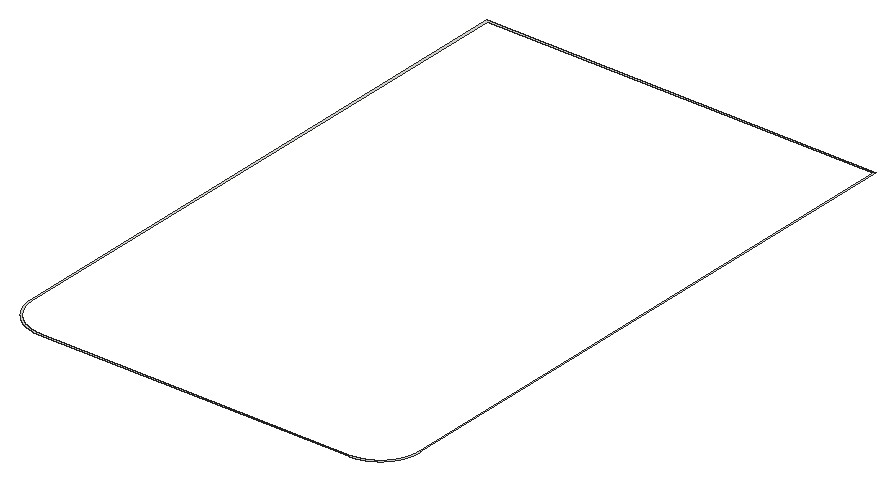
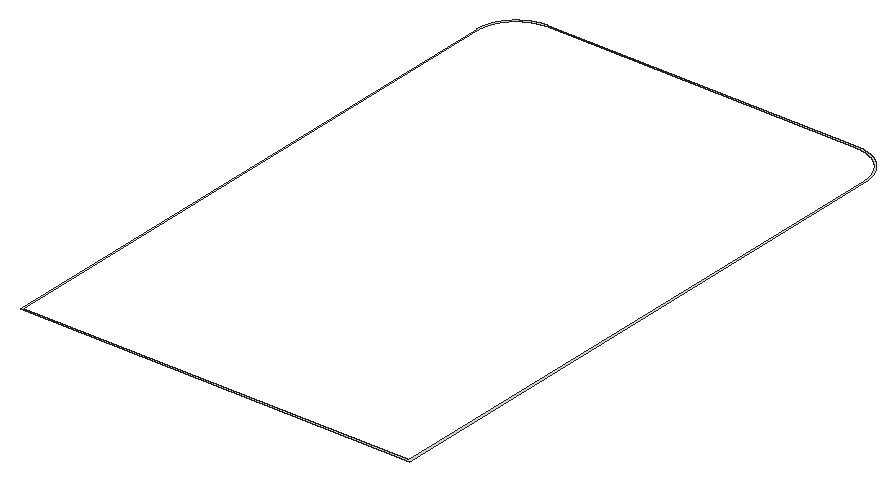
# SketchUp Ruby script. Lengths in inches.
U = 1.inch
M = Sketchup.active_model
def pt(a) = Geom::Point3d.new(a.map { |v| v * U })
def face(e, loops, mat)
  f = e.add_face(loops[0].map { |a| pt(a) })
  loops[1..].each { |l| e.add_face(l.map { |a| pt(a) }).erase! }
  f.material = f.back_material = mat if mat
  f
end
# faces: each face lists its corners as indices into pts; further lists are holes
def faces(e, pts, list, mat = nil) = list.each { |f| face(e, (f[0].is_a?(Array) ? f : [f]).map { |l| l.map { |i| pts[i] } }, mat) }
# xy, xz, yz: faces in a plane at the given z, y or x. An outline is a flat list of corners, or four numbers for a rectangle; further outlines are holes
def ring(l) = l.size == 4 ? [[l[0], l[1]], [l[2], l[1]], [l[2], l[3]], [l[0], l[3]]] : l.each_slice(2).to_a
def flat(e, list, mat, &to3) = list.each { |f| face(e, (f[0].is_a?(Array) ? f : [f]).map { |l| ring(l).map { |u, v| to3.(u, v) } }, mat) }
def xy(e, z, list, mat = nil) = flat(e, list, mat) { |x, y| [x, y, z] }
def xz(e, y, list, mat = nil) = flat(e, list, mat) { |x, z| [x, y, z] }
def yz(e, x, list, mat = nil) = flat(e, list, mat) { |y, z| [x, y, z] }
def lines(e, pts, list) = list.each { |a, b| e.add_line(pt(pts[a]), pt(pts[b])) }
# prism: a flat outline (further loops are holes) pulled along v
def prism(e, loops, v, mat = nil)
  f = face(e, loops, mat); d = Geom::Vector3d.new(v.map { |x| x * U })
  f.pushpull(f.normal.samedirection?(d) ? d.length : -d.length)
end
def box(e, o, s, mat = nil) = prism(e, [[o, [o[0] + s[0], o[1], o[2]], [o[0] + s[0], o[1] + s[1], o[2]], [o[0], o[1] + s[1], o[2]]]], [0, 0, s[2]], mat)
def at(x, y, z, deg = 0) = Geom::Transformation.translation(pt([x, y, z])) * Geom::Transformation.rotation(ORIGIN, Z_AXIS, deg.degrees)
def axes(o, x, y, z) = Geom::Transformation.new([*x, 0, *y, 0, *z, 0, *pt(o).to_a, 1])
def part(name) = M.definitions.add(name)
# library, detail: a bought-in or finely detailed component or shape, given as its bounding box
def library(name, o, s) = part(name).tap { |d| box(d.entities, o, s) }
def detail(e, o, s) = box(e.add_group.entities, o, s)
def put(e, d, t, mat = nil) = e.add_instance(d, t).tap { |i| i.material = mat if mat }
def group(e, t, mat = nil) = e.add_group.tap { |g| g.transformation = t; g.material = mat if mat }.entities
root = M.entities
xy(root,349.5,[[[38.61,204,270.39,204,270.79,204.01,271.18,204.02,271.57,204.04,271.96,204.0625,272.35,204.09,272.75,204.125,273.14,204.16,273.92,204.26,274.3,204.31,275.08,204.43,275.47,204.5,275.85,204.58,276.24,204.66,276.62,204.74,277.38,204.92,277.76,205.02,278.14,205.125,278.52,205.24,278.9,205.35,279.64,205.59,280.38,205.85,280.75,205.99,281.12,206.14,281.48,206.28,281.84,206.4375,282.2,206.59,282.56,206.76,282.92,206.92,283.27,207.09,283.97,207.45,284.31,207.64,284.66,207.83,285,208.02,285.34,208.22,285.67,208.42,286.01,208.63,286.34,208.84,286.67,209.06,286.99,209.28,287.3125,209.5,287.63,209.73,287.95,209.96,288.57,210.44,288.88,210.6875,289.18,210.93,289.48,211.1875,289.78,211.44,290.07,211.71,290.36,211.97,290.65,212.24,290.93,212.51,291.49,213.07,291.76,213.35,292.03,213.64,292.29,213.93,292.56,214.22,292.8125,214.52,293.07,214.82,293.3125,215.12,293.56,215.43,294.04,216.05,294.27,216.37,294.5,216.6875,294.72,217.01,294.94,217.33,295.16,217.66,295.37,217.99,295.58,218.33,295.78,218.66,295.98,219,296.17,219.34,296.36,219.69,296.55,220.03,296.91,220.73,297.08,221.08,297.24,221.44,297.41,221.8,297.5625,222.16,297.72,222.52,297.86,222.88,298.01,223.25,298.15,223.62,298.41,224.36,298.65,225.1,298.76,225.48,298.875,225.86,298.98,226.24,299.08,226.62,299.26,227.38,299.34,227.76,299.42,228.15,299.5,228.53,299.57,228.92,299.69,229.7,299.74,230.08,299.84,230.86,299.875,231.25,299.91,231.65,299.9375,232.04,299.96,232.43,299.98,232.82,299.99,233.21,300,233.61,300,660,9,660,9,233.61,9.01,233.21,9.02,232.82,9.04,232.43,9.0625,232.04,9.09,231.65,9.125,231.25,9.16,230.86,9.26,230.08,9.31,229.7,9.43,228.92,9.5,228.53,9.58,228.15,9.66,227.76,9.74,227.38,9.92,226.62,10.02,226.24,10.125,225.86,10.24,225.48,10.35,225.1,10.59,224.36,10.85,223.62,10.99,223.25,11.14,222.88,11.28,222.52,11.4375,222.16,11.59,221.8,11.76,221.44,11.92,221.08,12.09,220.73,12.45,220.03,12.64,219.69,12.83,219.34,13.02,219,13.22,218.66,13.42,218.33,13.63,217.99,13.84,217.66,14.06,217.33,14.28,217.01,14.5,216.6875,14.73,216.37,14.96,216.05,15.44,215.43,15.6875,215.12,15.93,214.82,16.1875,214.52,16.44,214.22,16.71,213.93,16.97,213.64,17.24,213.35,17.51,213.07,18.07,212.51,18.35,212.24,18.64,211.97,18.93,211.71,19.22,211.44,19.52,211.1875,19.82,210.93,20.12,210.6875,20.43,210.44,21.05,209.96,21.37,209.73,21.6875,209.5,22.01,209.28,22.33,209.06,22.66,208.84,22.99,208.63,23.33,208.42,23.66,208.22,24,208.02,24.34,207.83,24.69,207.64,25.03,207.45,25.73,207.09,26.08,206.92,26.44,206.76,26.8,206.59,27.16,206.4375,27.52,206.28,27.88,206.14,28.25,205.99,28.62,205.85,29.36,205.59,30.1,205.35,30.48,205.24,30.86,205.125,31.24,205.02,31.62,204.92,32.38,204.74,32.76,204.66,33.15,204.58,33.53,204.5,33.92,204.43,34.7,204.31,35.08,204.26,35.86,204.16,36.25,204.125,36.65,204.09,37.04,204.0625,37.43,204.04,37.82,204.02,38.21,204.01],[38.62,205,37.86,205.02,37.48,205.04,37.1,205.0625,36.72,205.09,36.35,205.12,35.59,205.2,35.21,205.25,34.84,205.3,34.46,205.36,34.09,205.42,33.72,205.49,33.34,205.56,32.97,205.63,32.6,205.72,32.23,205.8,31.86,205.89,31.49,205.99,31.13,206.09,30.76,206.19,30.4,206.3,29.32,206.66,28.96,206.79,28.61,206.93,28.25,207.06,27.2,207.51,26.86,207.66,26.52,207.83,26.17,207.99,25.83,208.16,25.5,208.34,25.16,208.51,24.17,209.08,23.85,209.27,23.53,209.47,22.57,210.1,21.95,210.54,21.65,210.76,21.35,210.99,21.05,211.23,20.75,211.46,20.46,211.7,19.88,212.2,19.6,212.45,19.31,212.7,19.04,212.96,18.76,213.23,18.49,213.49,18.23,213.76,17.96,214.04,17.7,214.31,17.45,214.6,17.2,214.88,16.7,215.46,16.46,215.75,16.23,216.05,15.99,216.35,15.76,216.65,15.54,216.95,15.1,217.57,14.47,218.53,14.27,218.85,14.08,219.17,13.51,220.16,13.34,220.5,13.16,220.83,12.99,221.17,12.83,221.52,12.66,221.86,12.51,222.2,12.06,223.25,11.93,223.61,11.79,223.96,11.66,224.32,11.3,225.4,11.19,225.76,11.09,226.13,10.99,226.49,10.89,226.86,10.8,227.23,10.72,227.6,10.63,227.97,10.56,228.34,10.49,228.72,10.42,229.09,10.36,229.46,10.3,229.84,10.25,230.21,10.2,230.59,10.12,231.35,10.09,231.72,10.0625,232.1,10.04,232.48,10.02,232.86,10,233.62,10,659,299,659,299,233.62,298.98,232.86,298.96,232.48,298.9375,232.1,298.91,231.72,298.88,231.35,298.8,230.59,298.75,230.21,298.7,229.84,298.64,229.46,298.58,229.09,298.51,228.72,298.44,228.34,298.37,227.97,298.28,227.6,298.2,227.23,298.11,226.86,298.01,226.49,297.91,226.13,297.81,225.76,297.7,225.4,297.34,224.32,297.21,223.96,297.07,223.61,296.94,223.25,296.49,222.2,296.34,221.86,296.17,221.52,296.01,221.17,295.84,220.83,295.66,220.5,295.49,220.16,294.92,219.17,294.73,218.85,294.53,218.53,293.9,217.57,293.46,216.95,293.24,216.65,293.01,216.35,292.77,216.05,292.54,215.75,292.3,215.46,291.8,214.88,291.55,214.6,291.3,214.31,291.04,214.04,290.77,213.76,290.51,213.49,290.24,213.23,289.96,212.96,289.69,212.7,289.4,212.45,289.12,212.2,288.54,211.7,288.25,211.46,287.95,211.23,287.65,210.99,287.35,210.76,287.05,210.54,286.43,210.1,285.47,209.47,285.15,209.27,284.83,209.08,283.84,208.51,283.5,208.34,283.17,208.16,282.83,207.99,282.48,207.83,282.14,207.66,281.8,207.51,280.75,207.06,280.39,206.93,280.04,206.79,279.68,206.66,278.6,206.3,278.24,206.19,277.87,206.09,277.51,205.99,277.14,205.89,276.77,205.8,276.4,205.72,276.03,205.63,275.66,205.56,275.28,205.49,274.91,205.42,274.54,205.36,274.16,205.3,273.79,205.25,273.41,205.2,272.65,205.12,272.28,205.09,271.9,205.0625,271.52,205.04,271.14,205.02,270.38,205]]])
